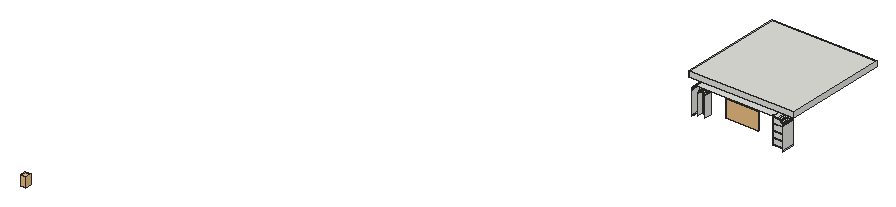
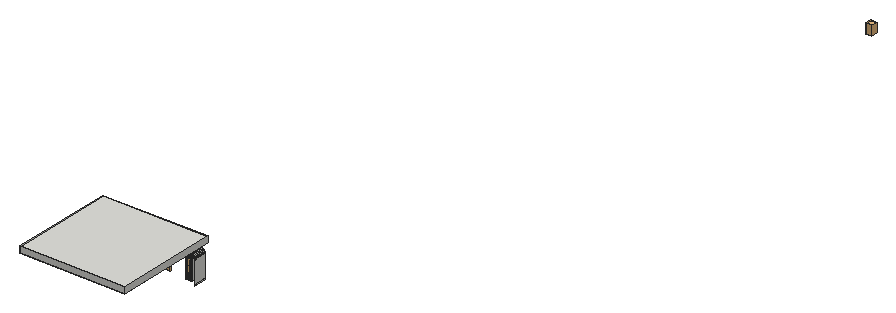
# SketchUp Ruby script. Lengths in inches.
U = 1.inch
M = Sketchup.active_model
def pt(a) = Geom::Point3d.new(a.map { |v| v * U })
def face(e, loops, mat)
  f = e.add_face(loops[0].map { |a| pt(a) })
  loops[1..].each { |l| e.add_face(l.map { |a| pt(a) }).erase! }
  f.material = f.back_material = mat if mat
  f
end
# faces: each face lists its corners as indices into pts; further lists are holes
def faces(e, pts, list, mat = nil) = list.each { |f| face(e, (f[0].is_a?(Array) ? f : [f]).map { |l| l.map { |i| pts[i] } }, mat) }
# xy, xz, yz: faces in a plane at the given z, y or x. An outline is a flat list of corners, or four numbers for a rectangle; further outlines are holes
def ring(l) = l.size == 4 ? [[l[0], l[1]], [l[2], l[1]], [l[2], l[3]], [l[0], l[3]]] : l.each_slice(2).to_a
def flat(e, list, mat, &to3) = list.each { |f| face(e, (f[0].is_a?(Array) ? f : [f]).map { |l| ring(l).map { |u, v| to3.(u, v) } }, mat) }
def xy(e, z, list, mat = nil) = flat(e, list, mat) { |x, y| [x, y, z] }
def xz(e, y, list, mat = nil) = flat(e, list, mat) { |x, z| [x, y, z] }
def yz(e, x, list, mat = nil) = flat(e, list, mat) { |y, z| [x, y, z] }
def lines(e, pts, list) = list.each { |a, b| e.add_line(pt(pts[a]), pt(pts[b])) }
# prism: a flat outline (further loops are holes) pulled along v
def prism(e, loops, v, mat = nil)
  f = face(e, loops, mat); d = Geom::Vector3d.new(v.map { |x| x * U })
  f.pushpull(f.normal.samedirection?(d) ? d.length : -d.length)
end
def box(e, o, s, mat = nil) = prism(e, [[o, [o[0] + s[0], o[1], o[2]], [o[0] + s[0], o[1] + s[1], o[2]], [o[0], o[1] + s[1], o[2]]]], [0, 0, s[2]], mat)
def at(x, y, z, deg = 0) = Geom::Transformation.translation(pt([x, y, z])) * Geom::Transformation.rotation(ORIGIN, Z_AXIS, deg.degrees)
def axes(o, x, y, z) = Geom::Transformation.new([*x, 0, *y, 0, *z, 0, *pt(o).to_a, 1])
def part(name) = M.definitions.add(name)
# library, detail: a bought-in or finely detailed component or shape, given as its bounding box
def library(name, o, s) = part(name).tap { |d| box(d.entities, o, s) }
def detail(e, o, s) = box(e.add_group.entities, o, s)
def put(e, d, t, mat = nil) = e.add_instance(d, t).tap { |i| i.material = mat if mat }
def group(e, t, mat = nil) = e.add_group.tap { |g| g.transformation = t; g.material = mat if mat }.entities
root = M.entities
M.materials.add("[0045_Goldenrod]1").color = [214, 181, 218]
M.materials.add("[Color G07]").color = [232, 230, 47]
c1 = library("Row of books",[-2.76,0,0],[10.13,7.78,9.38])
c2 = library("tv samsung",[0,6.14,2.62],[61.9,2.56,35.76])
c3 = library("0719lighting",[0,0,0],[19.69,19.69,39.41])
c4 = library("Group\#41",[0,0,0],[19.89,19.86,28.11])
c5 = library("9",[-32.42,-26.625,-4.37],[27.26,11.82,35.21])
c6 = library("Vase with flowers",[-1.1875,-2.53,0],[20.47,14.7,29.98])
c7 = library("Group\#45",[-0.79,0,0],[8.91,8.37,20.26])
c8 = library("FIFA+club+world+cup",[-109.48,-73.1,204.72],[11.79,11.96,20.26])
xy(root,41.1,[[185.773,11.1,200.205,37],[200.205,11.1,207.773,37]])
xy(root,42.1,[[185.773,11.1,207.773,37]])
xy(root,54.7,[[185.773,11.1,200.205,37],[200.205,11.1,207.773,37]])
xy(root,55.7,[[185.773,11.1,207.773,37]])
xy(root,68.3,[[185.773,11.1,200.205,37],[200.205,11.1,207.773,37]])
xy(root,69.3,[[185.773,11.1,207.773,37]])
xy(root,81.9,[[185.773,11.1,185.776,37],[185.776,11.1,200.209,37],[200.209,11.1,207.773,37]])
xy(root,82.9,[[185.773,11.1,185.776,37],[185.776,11.1,207.773,37]])
xy(root,95,[[185.773,11.1,196.463,37],[182.522,14.3125,183.773,15],[182.522,15,183.773,37],[25.222,30.3125,182.522,37]])
xy(root,96,[[25.222,11,196.463,37]])
xz(root,11.1,[[185.773,42.1,206.912,54.191],[185.773,55.7,206.912,67.791],[185.773,69.3,206.912,81.391],[185.773,82.9,185.773,94.491,195.602,94.491,197.078,94.395,198.529,94.106,199.93,93.631,201.257,92.976,202.487,92.154,203.599,91.179,204.574,90.067,205.396,88.837,206.051,87.51,206.526,86.109,206.815,84.658,206.912,83.182,206.93,82.9]])
xz(root,11.1,[[206.912,42.1,206.912,54.191,185.773,54.191,185.773,54.7,207.773,54.7,207.773,42.1],[206.912,55.7,206.912,67.791,185.773,67.791,185.773,68.3,207.773,68.3,207.773,55.7],[206.912,69.3,206.912,81.391,185.773,81.391,185.773,81.9,207.773,81.9,207.773,69.3],[206.93,82.9,206.912,83.182,206.815,84.658,206.526,86.109,206.051,87.51,205.396,88.837,204.574,90.067,203.599,91.179,202.487,92.154,201.257,92.976,199.93,93.631,198.529,94.106,197.078,94.395,195.602,94.491,185.773,94.491,185.773,95,196.463,95,197.939,94.903,199.39,94.615,200.791,94.139,202.118,93.485,203.348,92.663,204.46,91.6875,205.435,90.575,206.257,89.345,206.912,88.018,207.387,86.618,207.676,85.167,207.773,83.69,207.773,82.9]],"[Color G07]")
xz(root,14.3125,[[183.773,93.75,183.762,93.913,183.73,94.073,183.677,94.228,183.605,94.375,183.514,94.511,183.406,94.634,183.283,94.742,183.148,94.833,183.001,94.905,182.846,94.957,182.686,94.989,182.522,95,183.773,95]])
xz(root,30.3125,[[182.846,94.957,181.991,94.958,181.969,94.969,181.877,95,182.522,95,182.686,94.989],[180.896,94.958,26.222,95,181.014,95],[180.896,94.958,181.014,95,181.877,95,181.969,94.969,181.991,94.958],[181.014,95,181.104,95.032,181.321,95.071,181.542,95.074,181.76,95.039,181.877,95]])
xz(root,32.82,[[70.633,43.38,139.709,78.388]])
xz(root,37,[[185.773,41.1,207.773,42.1],[185.773,54.7,207.773,55.7],[185.773,68.3,207.773,69.3],[185.773,81.9,207.773,82.9]])
yz(root,13.856,[[11,38.224,37,84.634]])
yz(root,14.856,[[30.3125,38.224,37,84.634]])
yz(root,24.231,[[15,38.224,30.3125,80.163]])
yz(root,25.231,[[26.375,38.224,30.3125,80.097]])
yz(root,25.831,[[26.375,38.224,30.3125,80.097],[26.375,80.097,30.3125,82.605]])
yz(root,26.431,[[26.375,38.224,30.3125,80.097],[26.375,80.097,30.3125,83.614]])
yz(root,27.031,[[26.375,38.224,30.3125,80.097],[26.375,80.097,30.3125,84.34],[26.375,84.34,30.3125,84.373]])
yz(root,27.631,[[26.375,38.224,30.3125,80.097],[26.375,80.097,30.3125,84.833]])
yz(root,28.231,[[26.375,38.224,30.3125,80.097],[26.375,80.097,30.3125,85.293]])
yz(root,28.831,[[26.375,38.224,30.3125,80.097],[26.375,80.097,30.3125,85.542]])
yz(root,29.431,[[26.375,38.224,30.3125,80.097],[26.375,80.097,30.3125,85.79]])
yz(root,30.031,[[26.3125,38.224,30.3125,80.097],[26.3125,80.097,30.3125,85.939]])
yz(root,30.631,[[26.3125,38.224,30.3125,80.097],[26.3125,80.097,30.3125,86.018]])
yz(root,31.231,[[26.3125,38.224,30.3125,80.097],[26.3125,80.097,30.3125,86.097]])
yz(root,31.831,[[26.3125,38.224,30.3125,80.097],[26.3125,80.097,30.3125,86.018]])
yz(root,32.431,[[26.3125,38.224,30.3125,80.097],[26.3125,80.097,30.3125,85.939]])
yz(root,33.031,[[26.3125,38.224,30.3125,80.097],[26.3125,80.097,30.3125,85.79]])
yz(root,33.631,[[26.3125,38.224,30.3125,80.097],[26.3125,80.097,30.3125,85.542]])
yz(root,34.231,[[26.3125,38.224,30.3125,80.097],[26.3125,80.097,30.3125,85.293]])
yz(root,34.831,[[26.3125,38.224,30.3125,80.097],[26.3125,80.097,30.3125,84.833]])
yz(root,35.431,[[26.3125,38.224,30.3125,80.097],[26.3125,80.097,30.3125,84.34],[26.3125,84.34,30.3125,84.373]])
yz(root,36.031,[[26.3125,38.224,30.3125,80.097],[26.3125,80.097,30.3125,83.614]])
yz(root,36.631,[[26.3125,38.224,30.3125,80.097],[26.3125,80.097,30.3125,82.605]])
yz(root,38.231,[[15,38.224,30.3125,80.163]])
yz(root,185.773,[[11.1,42.1,37,54.7],[11.1,55.7,37,68.3],[11.1,69.3,37,81.9],[11.1,82.9,37,95]])
yz(root,207.773,[[11.1,36.567,37,41.1],[11.1,42.1,37,54.7],[11.1,55.7,37,68.3],[11.1,69.3,37,81.9],[11.1,82.9,37,83.69]])
yz(root,208.773,[[11,36.567,37,83.69]])
p = [[208.699,11,35.449],[208.699,37,35.449],[208.773,37,36.567],[208.773,11,36.567],[14.204,11,35.577],[13.943,11,36.889],
  [13.943,37,36.889],[14.204,37,35.577],[207.773,11.1,36.567],[207.773,37,36.567],[207.708,37,35.58],[207.708,11.1,35.58],
  [14.935,15,37.02],[15.17,15,35.836],[15.17,30.3125,35.836],[14.935,30.3125,37.02],[14.935,37,37.02],[15.17,37,35.836],
  [13.856,11,38.224],[13.856,37,38.224],[14.856,15,38.224],[14.856,30.3125,38.224],[14.856,37,38.224],[25.231,30.3125,80.097],
  [25.435,30.3125,81.65],[25.435,26.375,81.65],[25.231,26.375,80.097],[24.461,15,81.911],[24.231,15,80.163],[24.231,30.3125,80.163],
  [24.461,30.3125,81.911],[38.231,15,80.163],[38.001,15,81.911],[38.001,30.3125,81.911],[38.231,30.3125,80.163],[25.831,30.3125,82.605],
  [25.831,26.375,82.605],[24.907,15,82.988],[24.907,30.3125,82.988],[37.555,15,82.988],[37.555,30.3125,82.988],[36.427,30.3125,83.097],
  [36.631,30.3125,82.605],[36.631,26.3125,82.605],[36.427,26.3125,83.097],[25.161,15,83.602],[25.161,30.3125,83.602],[37.301,15,83.602],
  [37.301,30.3125,83.602],[36.031,30.3125,83.614],[36.031,26.3125,83.614],[25.638,15,84.222],[25.638,30.3125,84.222],[36.824,15,84.222],
  [36.824,30.3125,84.222],[26.431,30.3125,83.614],[26.988,30.3125,84.34],[26.988,26.375,84.34],[26.431,26.375,83.614],[208.773,11,83.69],
  [208.773,37,83.69],[208.667,37,85.297],[208.667,11,85.297],[207.676,11.1,85.167],[207.676,37,85.167],[207.773,37,83.69],
  [207.773,11.1,83.69],[26.275,15,85.053],[26.275,30.3125,85.053],[36.187,15,85.053],[36.187,30.3125,85.053],[27.031,30.3125,84.373],
  [27.031,26.375,84.373],[34.831,30.3125,84.833],[35.431,30.3125,84.373],[35.431,26.3125,84.373],[34.831,26.3125,84.833],[13.856,11,84.634],
  [13.953,11,86.117],[13.953,37,86.117],[13.856,37,84.634],[14.856,30.3125,84.634],[14.856,37,84.634],[14.945,37,85.987],
  [14.945,30.3125,85.987],[27.631,30.3125,84.833],[28.231,30.3125,85.293],[28.231,26.375,85.293],[27.631,26.375,84.833],[26.422,15,85.166],
  [26.422,30.3125,85.166],[36.04,15,85.166],[36.04,30.3125,85.166],[207.387,11.1,86.618],[207.387,37,86.618],[27.022,15,85.626],
  [27.022,30.3125,85.626],[35.44,15,85.626],[35.44,30.3125,85.626],[208.353,37,86.876],[208.353,11,86.876],[33.631,30.3125,85.542],
  [34.231,30.3125,85.293],[34.231,26.3125,85.293],[33.631,26.3125,85.542],[28.831,30.3125,85.542],[29.431,30.3125,85.79],[29.431,26.375,85.79],
  [28.831,26.375,85.542],[27.727,15,86.167],[27.727,30.3125,86.167],[34.735,15,86.167],[34.735,30.3125,86.167],[32.784,30.3125,85.893],
  [33.031,30.3125,85.79],[33.031,26.3125,85.79],[32.784,26.3125,85.893],[30.031,30.3125,85.939],[30.631,30.3125,86.018],[30.631,26.3125,86.018],
  [30.031,26.3125,85.939],[32.431,30.3125,85.939],[32.431,26.3125,85.939],[31.231,30.3125,86.097],[31.831,30.3125,86.018],[31.831,26.3125,86.018],
  [31.231,26.3125,86.097],[15.209,37,87.317],[15.209,30.3125,87.317],[14.243,11,87.576],[14.243,37,87.576],[28.448,15,86.466],
  [28.448,30.3125,86.466],[34.014,15,86.466],[34.014,30.3125,86.466],[29.048,15,86.714],[29.048,30.3125,86.714],[33.414,15,86.714],
  [33.414,30.3125,86.714],[206.912,11.1,88.018],[206.912,37,88.018],[29.417,15,86.867],[29.417,30.3125,86.867],[33.045,15,86.867],
  [33.045,30.3125,86.867],[207.836,37,88.401],[207.836,11,88.401],[29.9,15,86.931],[29.9,30.3125,86.931],[30.5,15,87.01],
  [30.5,30.3125,87.01],[32.561,15,86.931],[31.961,15,87.01],[31.961,30.3125,87.01],[32.561,30.3125,86.931],[31.231,15,87.106],
  [31.231,30.3125,87.106],[15.645,37,88.601],[15.645,30.3125,88.601],[14.721,11,88.984],[14.721,37,88.984],[206.257,11.1,89.345],
  [206.257,37,89.345],[207.123,37,89.845],[207.123,11,89.845],[16.245,37,89.817],[16.245,30.3125,89.817],[15.379,11,90.317],
  [15.379,37,90.317],[205.435,11.1,90.575],[205.435,37,90.575],[206.229,37,91.184],[206.229,11,91.184],[16.998,37,90.944],
  [16.998,30.3125,90.944],[16.205,11,91.553],[16.205,37,91.553],[204.46,11.1,91.6875],[204.46,37,91.6875],[17.892,37,91.964],
  [17.892,30.3125,91.964],[205.167,37,92.395],[205.167,11,92.395],[17.185,11,92.671],[17.185,37,92.671],[203.348,11.1,92.663],
  [203.348,37,92.663],[18.912,37,92.858],[18.912,30.3125,92.858],[203.957,37,93.456],[203.957,11,93.456],[18.303,11,93.651],
  [18.303,37,93.651],[202.118,11.1,93.485],[202.118,37,93.485],[20.039,37,93.611],[20.039,30.3125,93.611],[202.618,37,94.351],
  [202.618,11,94.351],[200.791,11.1,94.139],[200.791,37,94.139],[21.255,37,94.211],[21.255,30.3125,94.211],[19.539,11,94.477],
  [19.539,37,94.477],[183.762,14.3125,93.913],[183.773,14.3125,93.75],[183.773,30.3125,93.75],[183.762,30.3125,93.913],[183.73,14.3125,94.073],
  [183.73,30.3125,94.073],[199.39,11.1,94.615],[199.39,37,94.615],[183.677,14.3125,94.228],[183.677,30.3125,94.228],[183.605,14.3125,94.375],
  [183.605,30.3125,94.375],[22.539,37,94.647],[22.539,30.3125,94.647],[201.174,37,95.063],[201.174,11,95.063],[183.514,14.3125,94.511],
  [183.514,30.3125,94.511],[20.872,11,95.135],[20.872,37,95.135],[183.406,14.3125,94.634],[183.406,30.3125,94.634],[197.939,11.1,94.903],
  [197.939,37,94.903],[183.283,14.3125,94.742],[183.283,30.3125,94.742],[23.869,37,94.911],[23.869,30.3125,94.911],[183.148,14.3125,94.833],
  [183.148,30.3125,94.833],[183.001,14.3125,94.905],[183.001,30.3125,94.905],[196.463,11.1,95],[196.463,37,95],[182.846,14.3125,94.957],
  [182.846,30.3125,94.957],[25.222,37,95],[25.222,31.87,95],[25.222,30.3125,95],[182.522,14.3125,95],[182.686,14.3125,94.989],
  [182.686,30.3125,94.989],[182.522,30.3125,95],[182.522,15,95],[26.218,30.3125,95],[182.846,31.87,94.957],[181.991,30.3125,94.958],
  [180.896,30.3125,94.958],[26.222,30.3125,95],[22.28,11,95.613],[22.28,37,95.613],[199.649,37,95.581],[199.649,11,95.581],
  [23.738,11,95.903],[23.738,37,95.903],[198.07,37,95.895],[198.07,11,95.895],[25.222,11,96],[25.222,37,96],
  [196.463,37,96],[196.463,11,96],[29.431,15,85.79],[29.431,15,85.893],[207.773,15,82.9],[207.776,15,82.9],
  [207.773,15,81.9],[207.776,15,81.9],[184.915,11.1,81.391],[185.773,11.1,81.391],[184.912,11.1,94.491],[185.773,11.1,94.491],
  [184.912,11.1,67.791],[185.773,11.1,67.791],[184.912,11.1,54.191],[185.773,11.1,54.191],[206.912,11.1,69.3],[206.912,11.1,68.791],
  [206.912,11.1,42.1],[206.912,11.1,41.591],[206.912,11.1,55.7],[206.912,11.1,55.191]]
faces(root,p,[[0,1,2,3],[4,5,6,7],[8,9,10,11],[12,13,14,15],[16,15,14,17],[5,18,19,6],[20,12,15,21],[22,21,15,16],
  [23,24,25,26],[27,28,29,30],[31,32,33,34],[24,35,36,25],[37,27,30,38],[32,39,40,33],[41,42,43,44],[45,37,38,46],
  [39,47,48,40],[49,41,44,50],[51,45,46,52],[47,53,54,48],[55,56,57,58],[59,60,61,62],[63,64,65,66],[67,51,52,68],
  [53,69,70,54],[56,71,72,57],[73,74,75,76],[77,78,79,80],[81,82,83,84],[85,86,87,88],[89,67,68,90],[69,91,92,70],
  [93,94,64,63],[95,89,90,96],[91,97,98,92],[62,61,99,100],[101,102,103,104],[105,106,107,108],[109,95,96,110],[97,111,112,98],
  [113,114,115,116],[117,118,119,120],[121,113,116,122],[123,124,125,126],[84,83,127,128],[78,129,130,79],[131,109,110,132],[111,133,134,112],
  [135,131,132,136],[133,137,138,134],[139,140,94,93],[141,135,136,142],[137,143,144,138],[100,99,145,146],[147,141,142,148],[149,147,148,150],
  [151,152,153,154],[143,151,154,144],[155,149,150,156],[152,155,156,153],[128,127,157,158],[129,159,160,130],[161,162,140,139],[146,145,163,164],
  [158,157,165,166],[159,167,168,160],[169,170,162,161],[164,163,171,172],[166,165,173,174],[167,175,176,168],[177,178,170,169],[174,173,179,180],
  [172,171,181,182],[175,183,184,176],[185,186,178,177],[180,179,187,188],[182,181,189,190],[183,191,192,184],[193,194,186,185],[188,187,195,196],
  [190,189,197,198],[199,200,194,193],[196,195,201,202],[191,203,204,192],[205,206,207,208],[209,205,208,210],[211,212,200,199],[213,209,210,214],
  [215,213,214,216],[202,201,217,218],[198,197,219,220],[221,215,216,222],[203,223,224,204],[225,221,222,226],[227,228,212,211],[229,225,226,230],
  [218,217,231,232],[233,229,230,234],[235,233,234,236],[237,238,228,227],[239,235,236,240],[232,231,241,242,243],[244,245,246,247,248],[245,239,240,246],
  [223,254,255,224],[220,219,256,257],[254,258,259,255],[257,256,260,261],[258,262,263,259],[261,260,264,265]])
faces(root,p,[[249,243,242,250,240,251,252,253]],"[Color G07]")
lines(root,p,[[266,267],[268,269],[270,271],[272,273],[274,275],[276,277],[278,279],[280,281],[282,283],[284,285]])
put(root,c1,axes([192.26,24.18,42.1],[1.2198,0,0],[0,1,0],[0,0,1]))
put(root,c2,axes([140.21,39.02,39.75],[-1.1322,0,0],[0,-1,0],[0,0,1.0201]))
put(root,c3,axes([30.03,30.3125,54.21],[0.2475,0,0],[0,0.2475,0],[0,0,0.3267]))
put(root,c4,axes([197.09,28.36,55.49],[0.20368,0,0],[0,0.20368,0],[0,0,0.20368]))
put(root,c5,axes([198.4,37.2,56.65],[0.21794,0,0],[0,0.21794,0],[0,0,0.21794]))
put(root,c3,axes([30.03,30.3125,67.22],[0.2475,0,0],[0,0.2475,0],[0,0,0.3267]))
put(root,c6,axes([191.22,29.35,69.3],[0.4012,0,0],[0,0.4012,0],[0,0,0.4012]))
put(root,c7,axes([197.33,33.15,82.9],[-0.37332,-0.07095,0],[0.07095,-0.37332,0],[0,0,0.38]))
g1 = group(root,at(9,10,120))
xy(g1,-12,[[[0,0,222,221],[24,24,198,197]],[[24,24,198,197],[42,42,180,179]],[46,46,176,175]])
xy(g1,-12,[[[42,42,180,179],[46,46,176,175]]],"[0045_Goldenrod]1")
xy(g1,0,[[0,0,222,221]])
xz(g1,0,[[0,-12,222,0]])
xz(g1,221,[[0,-12,222,0]])
yz(g1,0,[[0,-12,221,0]])
yz(g1,222,[[0,-12,221,0]])
put(root,c8,at(-413.26,-1033.02,0))
